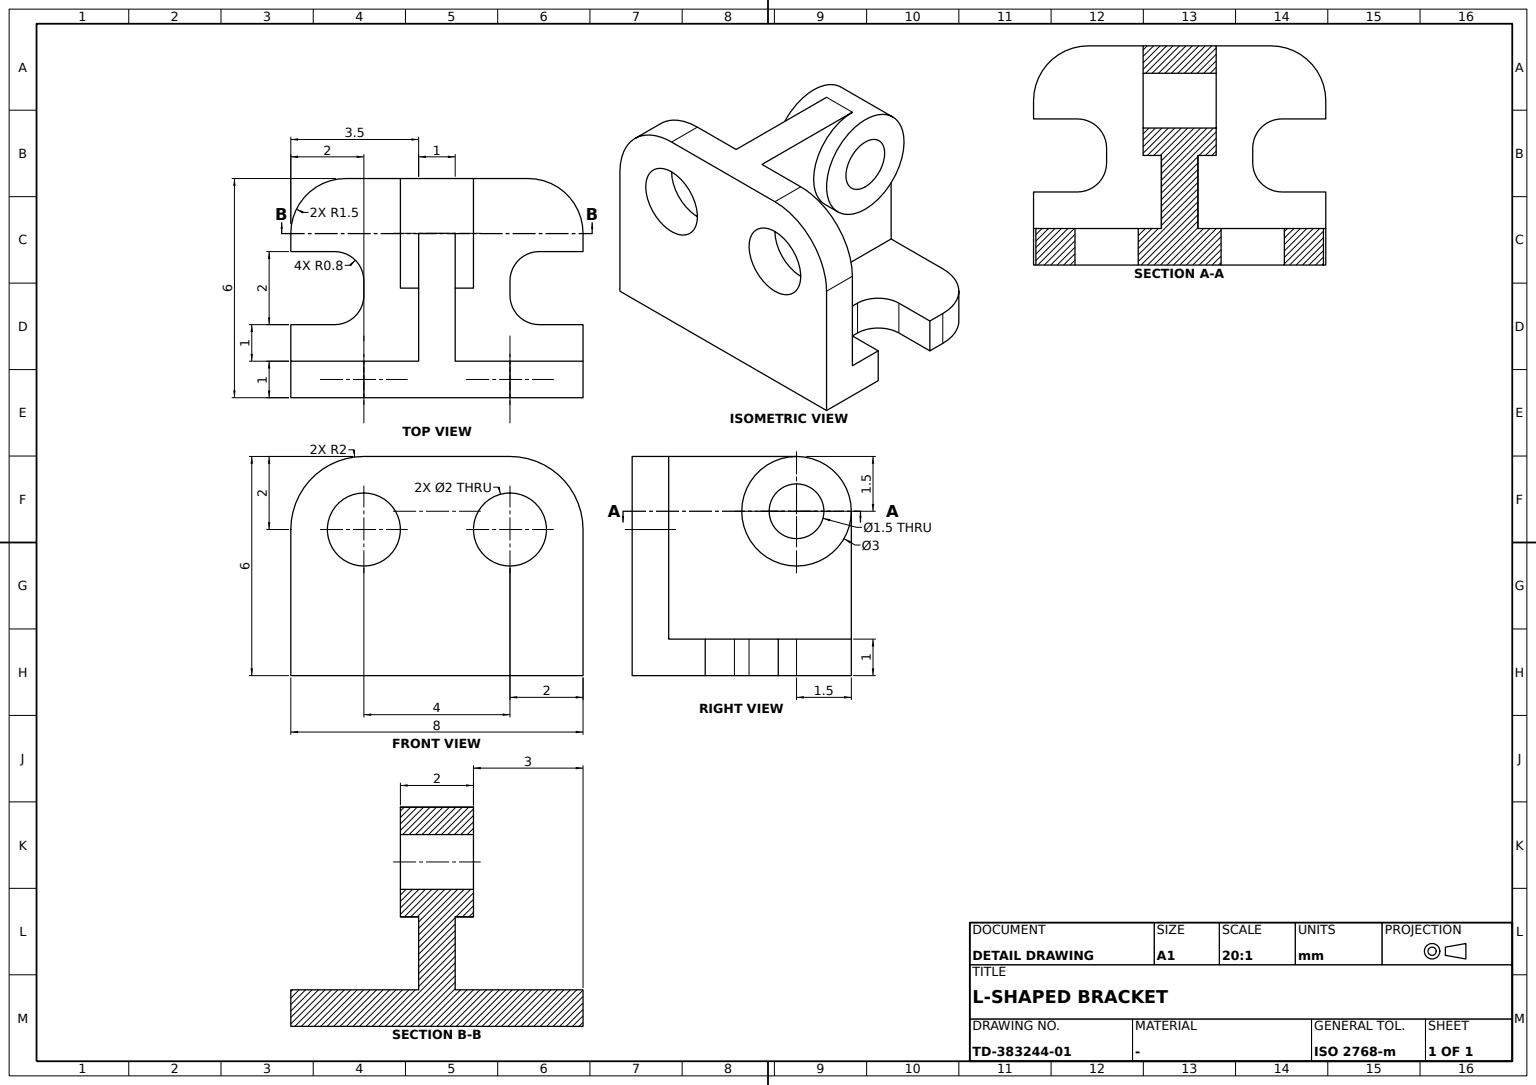
ISO-10303-21;
HEADER;
FILE_DESCRIPTION((''),'2;1');
FILE_NAME('','',(''),(''),'','','');
FILE_SCHEMA(('AUTOMOTIVE_DESIGN'));
ENDSEC;
DATA;
#1=APPLICATION_CONTEXT('');
#2=PRODUCT_CONTEXT('',#1,'mechanical');
#3=PRODUCT('','','',(#2));
#4=PRODUCT_DEFINITION_FORMATION('','',#3);
#5=PRODUCT_DEFINITION_CONTEXT('',#1,'design');
#6=PRODUCT_DEFINITION('','',#4,#5);
#7=PRODUCT_DEFINITION_SHAPE('','',#6);
#8=(LENGTH_UNIT()NAMED_UNIT(*)SI_UNIT(.MILLI.,.METRE.));
#9=(NAMED_UNIT(*)PLANE_ANGLE_UNIT()SI_UNIT($,.RADIAN.));
#10=(NAMED_UNIT(*)SI_UNIT($,.STERADIAN.)SOLID_ANGLE_UNIT());
#11=UNCERTAINTY_MEASURE_WITH_UNIT(LENGTH_MEASURE(0.005),#8,'distance_accuracy_value','');
#12=(GEOMETRIC_REPRESENTATION_CONTEXT(3)GLOBAL_UNCERTAINTY_ASSIGNED_CONTEXT((#11))GLOBAL_UNIT_ASSIGNED_CONTEXT((#8,#9,#10))REPRESENTATION_CONTEXT('',''));
#13=CARTESIAN_POINT('',(-2.,0.2,0.));
#14=VERTEX_POINT('',#13);
#15=CARTESIAN_POINT('',(-2.,-0.2,0.));
#16=VERTEX_POINT('',#15);
#17=CARTESIAN_POINT('',(-2.,0.,0.));
#18=DIRECTION('',(0.,-1.,0.));
#19=VECTOR('',#18,1000.);
#20=LINE('',#17,#19);
#21=EDGE_CURVE('',#14,#16,#20,.T.);
#22=ORIENTED_EDGE('',*,*,#21,.T.);
#23=CARTESIAN_POINT('',(-2.,-0.2,1.));
#24=VERTEX_POINT('',#23);
#25=CARTESIAN_POINT('',(-2.,-0.2,0.5));
#26=DIRECTION('',(0.,0.,1.));
#27=VECTOR('',#26,1000.);
#28=LINE('',#25,#27);
#29=EDGE_CURVE('',#16,#24,#28,.T.);
#30=ORIENTED_EDGE('',*,*,#29,.T.);
#31=CARTESIAN_POINT('',(-2.,0.2,1.));
#32=VERTEX_POINT('',#31);
#33=CARTESIAN_POINT('',(-2.,0.,1.));
#34=LINE('',#33,#19);
#35=EDGE_CURVE('',#32,#24,#34,.T.);
#36=ORIENTED_EDGE('',*,*,#35,.F.);
#37=CARTESIAN_POINT('',(-2.,0.2,0.5));
#38=LINE('',#37,#27);
#39=EDGE_CURVE('',#14,#32,#38,.T.);
#40=ORIENTED_EDGE('',*,*,#39,.F.);
#41=EDGE_LOOP('',(#22,#30,#36,#40));
#42=FACE_BOUND('',#41,.T.);
#43=DIRECTION('',(-1.,0.,0.));
#44=AXIS2_PLACEMENT_3D('',#13,#43,#18);
#45=PLANE('',#44);
#46=ADVANCED_FACE('',(#42),#45,.T.);
#47=CARTESIAN_POINT('',(2.8,1.,0.));
#48=VERTEX_POINT('',#47);
#49=CARTESIAN_POINT('',(2.8,1.,1.));
#50=VERTEX_POINT('',#49);
#51=CARTESIAN_POINT('',(2.8,1.,0.5));
#52=LINE('',#51,#27);
#53=EDGE_CURVE('',#48,#50,#52,.T.);
#54=ORIENTED_EDGE('',*,*,#53,.F.);
#55=CARTESIAN_POINT('',(4.,1.,0.));
#56=VERTEX_POINT('',#55);
#57=CARTESIAN_POINT('',(-2.8,1.,0.));
#58=DIRECTION('',(1.,0.,0.));
#59=VECTOR('',#58,1000.);
#60=LINE('',#57,#59);
#61=EDGE_CURVE('',#48,#56,#60,.T.);
#62=ORIENTED_EDGE('',*,*,#61,.T.);
#63=CARTESIAN_POINT('',(4.,1.,1.));
#64=VERTEX_POINT('',#63);
#65=LINE('',#55,#27);
#66=EDGE_CURVE('',#56,#64,#65,.T.);
#67=ORIENTED_EDGE('',*,*,#66,.T.);
#68=CARTESIAN_POINT('',(-2.8,1.,1.));
#69=LINE('',#68,#59);
#70=EDGE_CURVE('',#50,#64,#69,.T.);
#71=ORIENTED_EDGE('',*,*,#70,.F.);
#72=EDGE_LOOP('',(#54,#62,#67,#71));
#73=FACE_BOUND('',#72,.T.);
#74=DIRECTION('',(0.,1.,0.));
#75=AXIS2_PLACEMENT_3D('',#57,#74,#43);
#76=PLANE('',#75);
#77=ADVANCED_FACE('',(#73),#76,.F.);
#78=CARTESIAN_POINT('',(0.5,3.,1.));
#79=VERTEX_POINT('',#78);
#80=CARTESIAN_POINT('',(0.5,3.,4.5));
#81=VERTEX_POINT('',#80);
#82=CARTESIAN_POINT('',(0.5,3.,0.));
#83=LINE('',#82,#27);
#84=EDGE_CURVE('',#79,#81,#83,.T.);
#85=ORIENTED_EDGE('',*,*,#84,.F.);
#86=CARTESIAN_POINT('',(2.5,3.,1.));
#87=VERTEX_POINT('',#86);
#88=CARTESIAN_POINT('',(0.,3.,1.));
#89=LINE('',#88,#59);
#90=EDGE_CURVE('',#79,#87,#89,.T.);
#91=ORIENTED_EDGE('',*,*,#90,.T.);
#92=CARTESIAN_POINT('',(2.5,3.,0.));
#93=VERTEX_POINT('',#92);
#94=CARTESIAN_POINT('',(2.5,3.,0.5));
#95=LINE('',#94,#27);
#96=EDGE_CURVE('',#93,#87,#95,.T.);
#97=ORIENTED_EDGE('',*,*,#96,.F.);
#98=CARTESIAN_POINT('',(-2.5,3.,0.));
#99=VERTEX_POINT('',#98);
#100=CARTESIAN_POINT('',(0.,3.,0.));
#101=LINE('',#100,#59);
#102=EDGE_CURVE('',#99,#93,#101,.T.);
#103=ORIENTED_EDGE('',*,*,#102,.F.);
#104=CARTESIAN_POINT('',(-2.5,3.,1.));
#105=VERTEX_POINT('',#104);
#106=CARTESIAN_POINT('',(-2.5,3.,0.5));
#107=LINE('',#106,#27);
#108=EDGE_CURVE('',#99,#105,#107,.T.);
#109=ORIENTED_EDGE('',*,*,#108,.T.);
#110=CARTESIAN_POINT('',(-0.5,3.,1.));
#111=VERTEX_POINT('',#110);
#112=EDGE_CURVE('',#105,#111,#89,.T.);
#113=ORIENTED_EDGE('',*,*,#112,.T.);
#114=CARTESIAN_POINT('',(-0.5,3.,4.5));
#115=VERTEX_POINT('',#114);
#116=CARTESIAN_POINT('',(-0.5,3.,0.));
#117=LINE('',#116,#27);
#118=EDGE_CURVE('',#111,#115,#117,.T.);
#119=ORIENTED_EDGE('',*,*,#118,.T.);
#120=CARTESIAN_POINT('',(0.,3.,4.5));
#121=LINE('',#120,#59);
#122=EDGE_CURVE('',#115,#81,#121,.T.);
#123=ORIENTED_EDGE('',*,*,#122,.T.);
#124=EDGE_LOOP('',(#85,#91,#97,#103,#109,#113,#119,#123));
#125=FACE_BOUND('',#124,.T.);
#126=AXIS2_PLACEMENT_3D('',#98,#18,#58);
#127=PLANE('',#126);
#128=ADVANCED_FACE('',(#125),#127,.F.);
#129=CARTESIAN_POINT('',(-2.8,-1.,0.));
#130=VERTEX_POINT('',#129);
#131=CARTESIAN_POINT('',(-4.,-1.,0.));
#132=VERTEX_POINT('',#131);
#133=CARTESIAN_POINT('',(0.,-1.,0.));
#134=VECTOR('',#43,1000.);
#135=LINE('',#133,#134);
#136=EDGE_CURVE('',#130,#132,#135,.T.);
#137=ORIENTED_EDGE('',*,*,#136,.F.);
#138=CARTESIAN_POINT('',(-2.8,-0.2,0.));
#139=AXIS2_PLACEMENT_3D('',#138,#26,#58);
#140=CIRCLE('',#139,0.8);
#141=EDGE_CURVE('',#130,#16,#140,.T.);
#142=ORIENTED_EDGE('',*,*,#141,.T.);
#143=ORIENTED_EDGE('',*,*,#21,.F.);
#144=VERTEX_POINT('',#57);
#145=CARTESIAN_POINT('',(-2.8,0.2,0.));
#146=AXIS2_PLACEMENT_3D('',#145,#26,#58);
#147=CIRCLE('',#146,0.8);
#148=EDGE_CURVE('',#14,#144,#147,.T.);
#149=ORIENTED_EDGE('',*,*,#148,.T.);
#150=CARTESIAN_POINT('',(-4.,1.,0.));
#151=VERTEX_POINT('',#150);
#152=CARTESIAN_POINT('',(0.,1.,0.));
#153=LINE('',#152,#134);
#154=EDGE_CURVE('',#144,#151,#153,.T.);
#155=ORIENTED_EDGE('',*,*,#154,.T.);
#156=CARTESIAN_POINT('',(-4.,1.5,0.));
#157=VERTEX_POINT('',#156);
#158=CARTESIAN_POINT('',(-4.,0.,0.));
#159=VECTOR('',#74,1000.);
#160=LINE('',#158,#159);
#161=EDGE_CURVE('',#151,#157,#160,.T.);
#162=ORIENTED_EDGE('',*,*,#161,.T.);
#163=CARTESIAN_POINT('',(-2.5,1.5,0.));
#164=AXIS2_PLACEMENT_3D('',#163,#26,#58);
#165=CIRCLE('',#164,1.5);
#166=EDGE_CURVE('',#99,#157,#165,.T.);
#167=ORIENTED_EDGE('',*,*,#166,.F.);
#168=ORIENTED_EDGE('',*,*,#102,.T.);
#169=CARTESIAN_POINT('',(4.,1.5,0.));
#170=VERTEX_POINT('',#169);
#171=CARTESIAN_POINT('',(2.5,1.5,0.));
#172=AXIS2_PLACEMENT_3D('',#171,#26,#58);
#173=CIRCLE('',#172,1.5);
#174=EDGE_CURVE('',#170,#93,#173,.T.);
#175=ORIENTED_EDGE('',*,*,#174,.F.);
#176=CARTESIAN_POINT('',(4.,0.,0.));
#177=LINE('',#176,#19);
#178=EDGE_CURVE('',#170,#56,#177,.T.);
#179=ORIENTED_EDGE('',*,*,#178,.T.);
#180=ORIENTED_EDGE('',*,*,#61,.F.);
#181=CARTESIAN_POINT('',(2.,0.2,0.));
#182=VERTEX_POINT('',#181);
#183=CARTESIAN_POINT('',(2.8,0.2,0.));
#184=AXIS2_PLACEMENT_3D('',#183,#26,#58);
#185=CIRCLE('',#184,0.8);
#186=EDGE_CURVE('',#48,#182,#185,.T.);
#187=ORIENTED_EDGE('',*,*,#186,.T.);
#188=CARTESIAN_POINT('',(2.,-0.2,0.));
#189=VERTEX_POINT('',#188);
#190=CARTESIAN_POINT('',(2.,0.,0.));
#191=LINE('',#190,#19);
#192=EDGE_CURVE('',#182,#189,#191,.T.);
#193=ORIENTED_EDGE('',*,*,#192,.T.);
#194=CARTESIAN_POINT('',(2.8,-1.,0.));
#195=VERTEX_POINT('',#194);
#196=CARTESIAN_POINT('',(2.8,-0.2,0.));
#197=AXIS2_PLACEMENT_3D('',#196,#26,#58);
#198=CIRCLE('',#197,0.8);
#199=EDGE_CURVE('',#189,#195,#198,.T.);
#200=ORIENTED_EDGE('',*,*,#199,.T.);
#201=CARTESIAN_POINT('',(4.,-1.,0.));
#202=VERTEX_POINT('',#201);
#203=LINE('',#129,#59);
#204=EDGE_CURVE('',#195,#202,#203,.T.);
#205=ORIENTED_EDGE('',*,*,#204,.T.);
#206=CARTESIAN_POINT('',(4.,-3.,0.));
#207=VERTEX_POINT('',#206);
#208=EDGE_CURVE('',#202,#207,#177,.T.);
#209=ORIENTED_EDGE('',*,*,#208,.T.);
#210=CARTESIAN_POINT('',(-4.,-3.,0.));
#211=VERTEX_POINT('',#210);
#212=CARTESIAN_POINT('',(0.,-3.,0.));
#213=LINE('',#212,#134);
#214=EDGE_CURVE('',#207,#211,#213,.T.);
#215=ORIENTED_EDGE('',*,*,#214,.T.);
#216=EDGE_CURVE('',#211,#132,#160,.T.);
#217=ORIENTED_EDGE('',*,*,#216,.T.);
#218=EDGE_LOOP('',(#137,#142,#143,#149,#155,#162,#167,#168,#175,#179,#180,#187,#193,#200,#205,#209,#215,#217));
#219=FACE_BOUND('',#218,.T.);
#220=CARTESIAN_POINT('',(0.,0.,0.));
#221=AXIS2_PLACEMENT_3D('',#220,#26,#58);
#222=PLANE('',#221);
#223=ADVANCED_FACE('',(#219),#222,.F.);
#224=CARTESIAN_POINT('',(4.,1.5,1.));
#225=VERTEX_POINT('',#224);
#226=CARTESIAN_POINT('',(2.5,1.5,1.));
#227=AXIS2_PLACEMENT_3D('',#226,#26,#58);
#228=CIRCLE('',#227,1.5);
#229=EDGE_CURVE('',#225,#87,#228,.T.);
#230=ORIENTED_EDGE('',*,*,#229,.F.);
#231=CARTESIAN_POINT('',(4.,1.5,0.5));
#232=LINE('',#231,#27);
#233=EDGE_CURVE('',#170,#225,#232,.T.);
#234=ORIENTED_EDGE('',*,*,#233,.F.);
#235=ORIENTED_EDGE('',*,*,#174,.T.);
#236=ORIENTED_EDGE('',*,*,#96,.T.);
#237=EDGE_LOOP('',(#230,#234,#235,#236));
#238=FACE_BOUND('',#237,.T.);
#239=CARTESIAN_POINT('',(2.5,1.5,0.5));
#240=AXIS2_PLACEMENT_3D('',#239,#26,#58);
#241=CYLINDRICAL_SURFACE('',#240,1.5);
#242=ADVANCED_FACE('',(#238),#241,.T.);
#243=CARTESIAN_POINT('',(-1.,1.5,3.));
#244=VERTEX_POINT('',#243);
#245=CARTESIAN_POINT('',(-1.,1.5,4.5));
#246=DIRECTION('',(0.,0.,-1.));
#247=AXIS2_PLACEMENT_3D('',#245,#58,#246);
#248=CIRCLE('',#247,1.5);
#249=EDGE_CURVE('',#244,#244,#248,.T.);
#250=ORIENTED_EDGE('',*,*,#249,.F.);
#251=EDGE_LOOP('',(#250));
#252=FACE_BOUND('',#251,.T.);
#253=CARTESIAN_POINT('',(-1.,1.5,3.75));
#254=VERTEX_POINT('',#253);
#255=CIRCLE('',#247,0.75);
#256=EDGE_CURVE('',#254,#254,#255,.T.);
#257=ORIENTED_EDGE('',*,*,#256,.T.);
#258=EDGE_LOOP('',(#257));
#259=FACE_BOUND('',#258,.T.);
#260=CARTESIAN_POINT('',(-1.,0.,0.));
#261=AXIS2_PLACEMENT_3D('',#260,#58,#74);
#262=PLANE('',#261);
#263=ADVANCED_FACE('',(#252,#259),#262,.F.);
#264=CARTESIAN_POINT('',(4.,-3.,4.));
#265=VERTEX_POINT('',#264);
#266=CARTESIAN_POINT('',(4.,-2.,4.));
#267=VERTEX_POINT('',#266);
#268=CARTESIAN_POINT('',(4.,-2.5,4.));
#269=LINE('',#268,#19);
#270=EDGE_CURVE('',#265,#267,#269,.F.);
#271=ORIENTED_EDGE('',*,*,#270,.F.);
#272=LINE('',#206,#27);
#273=EDGE_CURVE('',#207,#265,#272,.T.);
#274=ORIENTED_EDGE('',*,*,#273,.F.);
#275=ORIENTED_EDGE('',*,*,#208,.F.);
#276=CARTESIAN_POINT('',(4.,-1.,1.));
#277=VERTEX_POINT('',#276);
#278=LINE('',#201,#27);
#279=EDGE_CURVE('',#202,#277,#278,.T.);
#280=ORIENTED_EDGE('',*,*,#279,.T.);
#281=CARTESIAN_POINT('',(4.,-2.,1.));
#282=VERTEX_POINT('',#281);
#283=CARTESIAN_POINT('',(4.,0.,1.));
#284=LINE('',#283,#19);
#285=EDGE_CURVE('',#277,#282,#284,.T.);
#286=ORIENTED_EDGE('',*,*,#285,.T.);
#287=CARTESIAN_POINT('',(4.,-2.,0.));
#288=VECTOR('',#246,1000.);
#289=LINE('',#287,#288);
#290=EDGE_CURVE('',#267,#282,#289,.T.);
#291=ORIENTED_EDGE('',*,*,#290,.F.);
#292=EDGE_LOOP('',(#271,#274,#275,#280,#286,#291));
#293=FACE_BOUND('',#292,.T.);
#294=AXIS2_PLACEMENT_3D('',#201,#43,#18);
#295=PLANE('',#294);
#296=ADVANCED_FACE('',(#293),#295,.F.);
#297=VERTEX_POINT('',#68);
#298=CARTESIAN_POINT('',(-2.8,0.2,1.));
#299=AXIS2_PLACEMENT_3D('',#298,#26,#58);
#300=CIRCLE('',#299,0.8);
#301=EDGE_CURVE('',#32,#297,#300,.T.);
#302=ORIENTED_EDGE('',*,*,#301,.T.);
#303=CARTESIAN_POINT('',(-2.8,1.,0.5));
#304=LINE('',#303,#27);
#305=EDGE_CURVE('',#144,#297,#304,.T.);
#306=ORIENTED_EDGE('',*,*,#305,.F.);
#307=ORIENTED_EDGE('',*,*,#148,.F.);
#308=ORIENTED_EDGE('',*,*,#39,.T.);
#309=EDGE_LOOP('',(#302,#306,#307,#308));
#310=FACE_BOUND('',#309,.T.);
#311=CARTESIAN_POINT('',(-2.8,0.2,0.5));
#312=AXIS2_PLACEMENT_3D('',#311,#26,#58);
#313=CYLINDRICAL_SURFACE('',#312,0.8);
#314=ADVANCED_FACE('',(#310),#313,.F.);
#315=CARTESIAN_POINT('',(0.5,-2.,1.));
#316=VERTEX_POINT('',#315);
#317=CARTESIAN_POINT('',(0.,-2.,1.));
#318=LINE('',#317,#134);
#319=EDGE_CURVE('',#282,#316,#318,.T.);
#320=ORIENTED_EDGE('',*,*,#319,.F.);
#321=ORIENTED_EDGE('',*,*,#285,.F.);
#322=CARTESIAN_POINT('',(2.8,-1.,1.));
#323=VERTEX_POINT('',#322);
#324=CARTESIAN_POINT('',(-2.8,-1.,1.));
#325=LINE('',#324,#59);
#326=EDGE_CURVE('',#323,#277,#325,.T.);
#327=ORIENTED_EDGE('',*,*,#326,.F.);
#328=CARTESIAN_POINT('',(2.,-0.2,1.));
#329=VERTEX_POINT('',#328);
#330=CARTESIAN_POINT('',(2.8,-0.2,1.));
#331=AXIS2_PLACEMENT_3D('',#330,#26,#58);
#332=CIRCLE('',#331,0.8);
#333=EDGE_CURVE('',#329,#323,#332,.T.);
#334=ORIENTED_EDGE('',*,*,#333,.F.);
#335=CARTESIAN_POINT('',(2.,0.2,1.));
#336=VERTEX_POINT('',#335);
#337=CARTESIAN_POINT('',(2.,0.,1.));
#338=LINE('',#337,#19);
#339=EDGE_CURVE('',#336,#329,#338,.T.);
#340=ORIENTED_EDGE('',*,*,#339,.F.);
#341=CARTESIAN_POINT('',(2.8,0.2,1.));
#342=AXIS2_PLACEMENT_3D('',#341,#26,#58);
#343=CIRCLE('',#342,0.8);
#344=EDGE_CURVE('',#50,#336,#343,.T.);
#345=ORIENTED_EDGE('',*,*,#344,.F.);
#346=ORIENTED_EDGE('',*,*,#70,.T.);
#347=EDGE_CURVE('',#225,#64,#284,.T.);
#348=ORIENTED_EDGE('',*,*,#347,.F.);
#349=ORIENTED_EDGE('',*,*,#229,.T.);
#350=ORIENTED_EDGE('',*,*,#90,.F.);
#351=CARTESIAN_POINT('',(0.5,0.,1.));
#352=LINE('',#351,#159);
#353=EDGE_CURVE('',#316,#79,#352,.T.);
#354=ORIENTED_EDGE('',*,*,#353,.F.);
#355=EDGE_LOOP('',(#320,#321,#327,#334,#340,#345,#346,#348,#349,#350,#354));
#356=FACE_BOUND('',#355,.T.);
#357=CARTESIAN_POINT('',(0.,0.,1.));
#358=AXIS2_PLACEMENT_3D('',#357,#26,#58);
#359=PLANE('',#358);
#360=ADVANCED_FACE('',(#356),#359,.T.);
#361=CARTESIAN_POINT('',(2.,-3.,5.));
#362=VERTEX_POINT('',#361);
#363=CARTESIAN_POINT('',(2.,-3.,4.));
#364=AXIS2_PLACEMENT_3D('',#363,#74,#26);
#365=CIRCLE('',#364,1.);
#366=EDGE_CURVE('',#362,#362,#365,.T.);
#367=ORIENTED_EDGE('',*,*,#366,.F.);
#368=EDGE_LOOP('',(#367));
#369=FACE_BOUND('',#368,.T.);
#370=CARTESIAN_POINT('',(2.,-2.,3.));
#371=VERTEX_POINT('',#370);
#372=CARTESIAN_POINT('',(2.,-2.,4.));
#373=AXIS2_PLACEMENT_3D('',#372,#18,#246);
#374=CIRCLE('',#373,1.);
#375=EDGE_CURVE('',#371,#371,#374,.F.);
#376=ORIENTED_EDGE('',*,*,#375,.T.);
#377=EDGE_LOOP('',(#376));
#378=FACE_BOUND('',#377,.T.);
#379=CARTESIAN_POINT('',(2.,-2.5,4.));
#380=AXIS2_PLACEMENT_3D('',#379,#74,#43);
#381=CYLINDRICAL_SURFACE('',#380,1.);
#382=ADVANCED_FACE('',(#369,#378),#381,.F.);
#383=ORIENTED_EDGE('',*,*,#326,.T.);
#384=ORIENTED_EDGE('',*,*,#279,.F.);
#385=ORIENTED_EDGE('',*,*,#204,.F.);
#386=CARTESIAN_POINT('',(2.8,-1.,0.5));
#387=LINE('',#386,#27);
#388=EDGE_CURVE('',#195,#323,#387,.T.);
#389=ORIENTED_EDGE('',*,*,#388,.T.);
#390=EDGE_LOOP('',(#383,#384,#385,#389));
#391=FACE_BOUND('',#390,.T.);
#392=AXIS2_PLACEMENT_3D('',#129,#74,#43);
#393=PLANE('',#392);
#394=ADVANCED_FACE('',(#391),#393,.T.);
#395=CARTESIAN_POINT('',(-4.,1.5,1.));
#396=VERTEX_POINT('',#395);
#397=CARTESIAN_POINT('',(-2.5,1.5,1.));
#398=AXIS2_PLACEMENT_3D('',#397,#26,#58);
#399=CIRCLE('',#398,1.5);
#400=EDGE_CURVE('',#105,#396,#399,.T.);
#401=ORIENTED_EDGE('',*,*,#400,.F.);
#402=ORIENTED_EDGE('',*,*,#108,.F.);
#403=ORIENTED_EDGE('',*,*,#166,.T.);
#404=CARTESIAN_POINT('',(-4.,1.5,0.5));
#405=LINE('',#404,#27);
#406=EDGE_CURVE('',#157,#396,#405,.T.);
#407=ORIENTED_EDGE('',*,*,#406,.T.);
#408=EDGE_LOOP('',(#401,#402,#403,#407));
#409=FACE_BOUND('',#408,.T.);
#410=CARTESIAN_POINT('',(-2.5,1.5,0.5));
#411=AXIS2_PLACEMENT_3D('',#410,#26,#58);
#412=CYLINDRICAL_SURFACE('',#411,1.5);
#413=ADVANCED_FACE('',(#409),#412,.T.);
#414=ORIENTED_EDGE('',*,*,#353,.T.);
#415=ORIENTED_EDGE('',*,*,#84,.T.);
#416=CARTESIAN_POINT('',(0.5,1.5,6.));
#417=VERTEX_POINT('',#416);
#418=CARTESIAN_POINT('',(0.5,1.5,4.5));
#419=AXIS2_PLACEMENT_3D('',#418,#58,#246);
#420=CIRCLE('',#419,1.5);
#421=EDGE_CURVE('',#417,#81,#420,.T.);
#422=ORIENTED_EDGE('',*,*,#421,.F.);
#423=CARTESIAN_POINT('',(0.5,-2.,6.));
#424=VERTEX_POINT('',#423);
#425=CARTESIAN_POINT('',(0.5,-3.,6.));
#426=LINE('',#425,#159);
#427=EDGE_CURVE('',#424,#417,#426,.T.);
#428=ORIENTED_EDGE('',*,*,#427,.F.);
#429=CARTESIAN_POINT('',(0.5,-2.,0.));
#430=LINE('',#429,#288);
#431=EDGE_CURVE('',#424,#316,#430,.T.);
#432=ORIENTED_EDGE('',*,*,#431,.T.);
#433=EDGE_LOOP('',(#414,#415,#422,#428,#432));
#434=FACE_BOUND('',#433,.T.);
#435=CARTESIAN_POINT('',(0.5,0.,0.));
#436=AXIS2_PLACEMENT_3D('',#435,#58,#74);
#437=PLANE('',#436);
#438=ADVANCED_FACE('',(#434),#437,.T.);
#439=CARTESIAN_POINT('',(-2.,-3.,5.));
#440=VERTEX_POINT('',#439);
#441=CARTESIAN_POINT('',(-2.,-3.,4.));
#442=AXIS2_PLACEMENT_3D('',#441,#74,#26);
#443=CIRCLE('',#442,1.);
#444=EDGE_CURVE('',#440,#440,#443,.T.);
#445=ORIENTED_EDGE('',*,*,#444,.T.);
#446=EDGE_LOOP('',(#445));
#447=FACE_BOUND('',#446,.T.);
#448=ORIENTED_EDGE('',*,*,#366,.T.);
#449=EDGE_LOOP('',(#448));
#450=FACE_BOUND('',#449,.T.);
#451=ORIENTED_EDGE('',*,*,#273,.T.);
#452=CARTESIAN_POINT('',(2.,-3.,6.));
#453=VERTEX_POINT('',#452);
#454=CIRCLE('',#364,2.);
#455=EDGE_CURVE('',#265,#453,#454,.F.);
#456=ORIENTED_EDGE('',*,*,#455,.T.);
#457=CARTESIAN_POINT('',(-2.,-3.,6.));
#458=VERTEX_POINT('',#457);
#459=CARTESIAN_POINT('',(4.,-3.,6.));
#460=LINE('',#459,#59);
#461=EDGE_CURVE('',#458,#453,#460,.T.);
#462=ORIENTED_EDGE('',*,*,#461,.F.);
#463=CARTESIAN_POINT('',(-4.,-3.,4.));
#464=VERTEX_POINT('',#463);
#465=CIRCLE('',#442,2.);
#466=EDGE_CURVE('',#458,#464,#465,.F.);
#467=ORIENTED_EDGE('',*,*,#466,.T.);
#468=LINE('',#210,#27);
#469=EDGE_CURVE('',#211,#464,#468,.T.);
#470=ORIENTED_EDGE('',*,*,#469,.F.);
#471=ORIENTED_EDGE('',*,*,#214,.F.);
#472=EDGE_LOOP('',(#451,#456,#462,#467,#470,#471));
#473=FACE_BOUND('',#472,.T.);
#474=AXIS2_PLACEMENT_3D('',#206,#74,#43);
#475=PLANE('',#474);
#476=ADVANCED_FACE('',(#447,#450,#473),#475,.F.);
#477=ORIENTED_EDGE('',*,*,#29,.F.);
#478=ORIENTED_EDGE('',*,*,#141,.F.);
#479=VERTEX_POINT('',#324);
#480=CARTESIAN_POINT('',(-2.8,-1.,0.5));
#481=LINE('',#480,#27);
#482=EDGE_CURVE('',#130,#479,#481,.T.);
#483=ORIENTED_EDGE('',*,*,#482,.T.);
#484=CARTESIAN_POINT('',(-2.8,-0.2,1.));
#485=AXIS2_PLACEMENT_3D('',#484,#26,#58);
#486=CIRCLE('',#485,0.8);
#487=EDGE_CURVE('',#479,#24,#486,.T.);
#488=ORIENTED_EDGE('',*,*,#487,.T.);
#489=EDGE_LOOP('',(#477,#478,#483,#488));
#490=FACE_BOUND('',#489,.T.);
#491=CARTESIAN_POINT('',(-2.8,-0.2,0.5));
#492=AXIS2_PLACEMENT_3D('',#491,#26,#58);
#493=CYLINDRICAL_SURFACE('',#492,0.8);
#494=ADVANCED_FACE('',(#490),#493,.F.);
#495=ORIENTED_EDGE('',*,*,#270,.T.);
#496=CARTESIAN_POINT('',(2.,-2.,6.));
#497=VERTEX_POINT('',#496);
#498=CIRCLE('',#373,2.);
#499=EDGE_CURVE('',#267,#497,#498,.T.);
#500=ORIENTED_EDGE('',*,*,#499,.T.);
#501=CARTESIAN_POINT('',(2.,-2.5,6.));
#502=LINE('',#501,#19);
#503=EDGE_CURVE('',#453,#497,#502,.F.);
#504=ORIENTED_EDGE('',*,*,#503,.F.);
#505=ORIENTED_EDGE('',*,*,#455,.F.);
#506=EDGE_LOOP('',(#495,#500,#504,#505));
#507=FACE_BOUND('',#506,.T.);
#508=AXIS2_PLACEMENT_3D('',#379,#18,#58);
#509=CYLINDRICAL_SURFACE('',#508,2.);
#510=ADVANCED_FACE('',(#507),#509,.T.);
#511=ORIENTED_EDGE('',*,*,#344,.T.);
#512=CARTESIAN_POINT('',(2.,0.2,0.5));
#513=LINE('',#512,#27);
#514=EDGE_CURVE('',#182,#336,#513,.T.);
#515=ORIENTED_EDGE('',*,*,#514,.F.);
#516=ORIENTED_EDGE('',*,*,#186,.F.);
#517=ORIENTED_EDGE('',*,*,#53,.T.);
#518=EDGE_LOOP('',(#511,#515,#516,#517));
#519=FACE_BOUND('',#518,.T.);
#520=CARTESIAN_POINT('',(2.8,0.2,0.5));
#521=AXIS2_PLACEMENT_3D('',#520,#26,#58);
#522=CYLINDRICAL_SURFACE('',#521,0.8);
#523=ADVANCED_FACE('',(#519),#522,.F.);
#524=CARTESIAN_POINT('',(-0.5,1.5,6.));
#525=VERTEX_POINT('',#524);
#526=CARTESIAN_POINT('',(0.,1.5,6.));
#527=LINE('',#526,#59);
#528=EDGE_CURVE('',#525,#417,#527,.T.);
#529=ORIENTED_EDGE('',*,*,#528,.T.);
#530=ORIENTED_EDGE('',*,*,#421,.T.);
#531=ORIENTED_EDGE('',*,*,#122,.F.);
#532=CARTESIAN_POINT('',(-0.5,1.5,4.5));
#533=AXIS2_PLACEMENT_3D('',#532,#58,#246);
#534=CIRCLE('',#533,1.5);
#535=EDGE_CURVE('',#525,#115,#534,.T.);
#536=ORIENTED_EDGE('',*,*,#535,.F.);
#537=EDGE_LOOP('',(#529,#530,#531,#536));
#538=FACE_BOUND('',#537,.T.);
#539=CARTESIAN_POINT('',(1.,1.5,3.));
#540=VERTEX_POINT('',#539);
#541=CARTESIAN_POINT('',(1.,1.5,4.5));
#542=AXIS2_PLACEMENT_3D('',#541,#58,#246);
#543=CIRCLE('',#542,1.5);
#544=EDGE_CURVE('',#540,#540,#543,.T.);
#545=ORIENTED_EDGE('',*,*,#544,.F.);
#546=EDGE_LOOP('',(#545));
#547=FACE_BOUND('',#546,.T.);
#548=ORIENTED_EDGE('',*,*,#249,.T.);
#549=EDGE_LOOP('',(#548));
#550=FACE_BOUND('',#549,.T.);
#551=CARTESIAN_POINT('',(0.,1.5,4.5));
#552=AXIS2_PLACEMENT_3D('',#551,#58,#74);
#553=CYLINDRICAL_SURFACE('',#552,1.5);
#554=ADVANCED_FACE('',(#538,#547,#550),#553,.T.);
#555=ORIENTED_EDGE('',*,*,#136,.T.);
#556=CARTESIAN_POINT('',(-4.,-1.,1.));
#557=VERTEX_POINT('',#556);
#558=LINE('',#131,#27);
#559=EDGE_CURVE('',#132,#557,#558,.T.);
#560=ORIENTED_EDGE('',*,*,#559,.T.);
#561=CARTESIAN_POINT('',(0.,-1.,1.));
#562=LINE('',#561,#134);
#563=EDGE_CURVE('',#479,#557,#562,.T.);
#564=ORIENTED_EDGE('',*,*,#563,.F.);
#565=ORIENTED_EDGE('',*,*,#482,.F.);
#566=EDGE_LOOP('',(#555,#560,#564,#565));
#567=FACE_BOUND('',#566,.T.);
#568=ADVANCED_FACE('',(#567),#393,.T.);
#569=ORIENTED_EDGE('',*,*,#154,.F.);
#570=ORIENTED_EDGE('',*,*,#305,.T.);
#571=CARTESIAN_POINT('',(-4.,1.,1.));
#572=VERTEX_POINT('',#571);
#573=CARTESIAN_POINT('',(0.,1.,1.));
#574=LINE('',#573,#134);
#575=EDGE_CURVE('',#297,#572,#574,.T.);
#576=ORIENTED_EDGE('',*,*,#575,.T.);
#577=LINE('',#150,#27);
#578=EDGE_CURVE('',#151,#572,#577,.T.);
#579=ORIENTED_EDGE('',*,*,#578,.F.);
#580=EDGE_LOOP('',(#569,#570,#576,#579));
#581=FACE_BOUND('',#580,.T.);
#582=ADVANCED_FACE('',(#581),#76,.F.);
#583=ORIENTED_EDGE('',*,*,#544,.T.);
#584=EDGE_LOOP('',(#583));
#585=FACE_BOUND('',#584,.T.);
#586=CARTESIAN_POINT('',(1.,1.5,3.75));
#587=VERTEX_POINT('',#586);
#588=CIRCLE('',#542,0.75);
#589=EDGE_CURVE('',#587,#587,#588,.T.);
#590=ORIENTED_EDGE('',*,*,#589,.F.);
#591=EDGE_LOOP('',(#590));
#592=FACE_BOUND('',#591,.T.);
#593=CARTESIAN_POINT('',(1.,0.,0.));
#594=AXIS2_PLACEMENT_3D('',#593,#58,#74);
#595=PLANE('',#594);
#596=ADVANCED_FACE('',(#585,#592),#595,.T.);
#597=ORIENTED_EDGE('',*,*,#118,.F.);
#598=CARTESIAN_POINT('',(-0.5,-2.,1.));
#599=VERTEX_POINT('',#598);
#600=CARTESIAN_POINT('',(-0.5,0.,1.));
#601=LINE('',#600,#159);
#602=EDGE_CURVE('',#599,#111,#601,.T.);
#603=ORIENTED_EDGE('',*,*,#602,.F.);
#604=CARTESIAN_POINT('',(-0.5,-2.,6.));
#605=VERTEX_POINT('',#604);
#606=CARTESIAN_POINT('',(-0.5,-2.,0.));
#607=LINE('',#606,#288);
#608=EDGE_CURVE('',#605,#599,#607,.T.);
#609=ORIENTED_EDGE('',*,*,#608,.F.);
#610=CARTESIAN_POINT('',(-0.5,-3.,6.));
#611=LINE('',#610,#159);
#612=EDGE_CURVE('',#605,#525,#611,.T.);
#613=ORIENTED_EDGE('',*,*,#612,.T.);
#614=ORIENTED_EDGE('',*,*,#535,.T.);
#615=EDGE_LOOP('',(#597,#603,#609,#613,#614));
#616=FACE_BOUND('',#615,.T.);
#617=CARTESIAN_POINT('',(-0.5,0.,0.));
#618=AXIS2_PLACEMENT_3D('',#617,#58,#74);
#619=PLANE('',#618);
#620=ADVANCED_FACE('',(#616),#619,.F.);
#621=ORIENTED_EDGE('',*,*,#578,.T.);
#622=CARTESIAN_POINT('',(-4.,0.,1.));
#623=LINE('',#622,#159);
#624=EDGE_CURVE('',#572,#396,#623,.T.);
#625=ORIENTED_EDGE('',*,*,#624,.T.);
#626=ORIENTED_EDGE('',*,*,#406,.F.);
#627=ORIENTED_EDGE('',*,*,#161,.F.);
#628=EDGE_LOOP('',(#621,#625,#626,#627));
#629=FACE_BOUND('',#628,.T.);
#630=AXIS2_PLACEMENT_3D('',#150,#58,#74);
#631=PLANE('',#630);
#632=ADVANCED_FACE('',(#629),#631,.F.);
#633=CARTESIAN_POINT('',(-2.,-2.,6.));
#634=VERTEX_POINT('',#633);
#635=LINE('',#633,#59);
#636=EDGE_CURVE('',#634,#605,#635,.T.);
#637=ORIENTED_EDGE('',*,*,#636,.F.);
#638=CARTESIAN_POINT('',(-2.,-2.5,6.));
#639=LINE('',#638,#19);
#640=EDGE_CURVE('',#458,#634,#639,.F.);
#641=ORIENTED_EDGE('',*,*,#640,.F.);
#642=ORIENTED_EDGE('',*,*,#461,.T.);
#643=ORIENTED_EDGE('',*,*,#503,.T.);
#644=EDGE_CURVE('',#424,#497,#635,.T.);
#645=ORIENTED_EDGE('',*,*,#644,.F.);
#646=ORIENTED_EDGE('',*,*,#427,.T.);
#647=ORIENTED_EDGE('',*,*,#528,.F.);
#648=ORIENTED_EDGE('',*,*,#612,.F.);
#649=EDGE_LOOP('',(#637,#641,#642,#643,#645,#646,#647,#648));
#650=FACE_BOUND('',#649,.T.);
#651=AXIS2_PLACEMENT_3D('',#457,#26,#58);
#652=PLANE('',#651);
#653=ADVANCED_FACE('',(#650),#652,.T.);
#654=ORIENTED_EDGE('',*,*,#66,.F.);
#655=ORIENTED_EDGE('',*,*,#178,.F.);
#656=ORIENTED_EDGE('',*,*,#233,.T.);
#657=ORIENTED_EDGE('',*,*,#347,.T.);
#658=EDGE_LOOP('',(#654,#655,#656,#657));
#659=FACE_BOUND('',#658,.T.);
#660=ADVANCED_FACE('',(#659),#295,.F.);
#661=ORIENTED_EDGE('',*,*,#256,.F.);
#662=EDGE_LOOP('',(#661));
#663=FACE_BOUND('',#662,.T.);
#664=ORIENTED_EDGE('',*,*,#589,.T.);
#665=EDGE_LOOP('',(#664));
#666=FACE_BOUND('',#665,.T.);
#667=CARTESIAN_POINT('',(-2.16,1.5,4.5));
#668=AXIS2_PLACEMENT_3D('',#667,#58,#74);
#669=CYLINDRICAL_SURFACE('',#668,0.75);
#670=ADVANCED_FACE('',(#663,#666),#669,.F.);
#671=CARTESIAN_POINT('',(-4.,-2.,1.));
#672=VERTEX_POINT('',#671);
#673=EDGE_CURVE('',#599,#672,#318,.T.);
#674=ORIENTED_EDGE('',*,*,#673,.T.);
#675=CARTESIAN_POINT('',(-4.,-2.,4.));
#676=VERTEX_POINT('',#675);
#677=CARTESIAN_POINT('',(-4.,-2.,0.));
#678=LINE('',#677,#27);
#679=EDGE_CURVE('',#672,#676,#678,.T.);
#680=ORIENTED_EDGE('',*,*,#679,.T.);
#681=CARTESIAN_POINT('',(-2.,-2.,4.));
#682=AXIS2_PLACEMENT_3D('',#681,#18,#246);
#683=CIRCLE('',#682,2.);
#684=EDGE_CURVE('',#634,#676,#683,.T.);
#685=ORIENTED_EDGE('',*,*,#684,.F.);
#686=ORIENTED_EDGE('',*,*,#636,.T.);
#687=ORIENTED_EDGE('',*,*,#608,.T.);
#688=EDGE_LOOP('',(#674,#680,#685,#686,#687));
#689=FACE_BOUND('',#688,.T.);
#690=CARTESIAN_POINT('',(-2.,-2.,3.));
#691=VERTEX_POINT('',#690);
#692=CIRCLE('',#682,1.);
#693=EDGE_CURVE('',#691,#691,#692,.F.);
#694=ORIENTED_EDGE('',*,*,#693,.F.);
#695=EDGE_LOOP('',(#694));
#696=FACE_BOUND('',#695,.T.);
#697=CARTESIAN_POINT('',(0.,-2.,0.));
#698=AXIS2_PLACEMENT_3D('',#697,#18,#58);
#699=PLANE('',#698);
#700=ADVANCED_FACE('',(#689,#696),#699,.F.);
#701=ORIENTED_EDGE('',*,*,#216,.F.);
#702=ORIENTED_EDGE('',*,*,#469,.T.);
#703=CARTESIAN_POINT('',(-4.,-2.5,4.));
#704=LINE('',#703,#19);
#705=EDGE_CURVE('',#464,#676,#704,.F.);
#706=ORIENTED_EDGE('',*,*,#705,.T.);
#707=ORIENTED_EDGE('',*,*,#679,.F.);
#708=EDGE_CURVE('',#672,#557,#623,.T.);
#709=ORIENTED_EDGE('',*,*,#708,.T.);
#710=ORIENTED_EDGE('',*,*,#559,.F.);
#711=EDGE_LOOP('',(#701,#702,#706,#707,#709,#710));
#712=FACE_BOUND('',#711,.T.);
#713=ADVANCED_FACE('',(#712),#631,.F.);
#714=ORIENTED_EDGE('',*,*,#575,.F.);
#715=ORIENTED_EDGE('',*,*,#301,.F.);
#716=ORIENTED_EDGE('',*,*,#35,.T.);
#717=ORIENTED_EDGE('',*,*,#487,.F.);
#718=ORIENTED_EDGE('',*,*,#563,.T.);
#719=ORIENTED_EDGE('',*,*,#708,.F.);
#720=ORIENTED_EDGE('',*,*,#673,.F.);
#721=ORIENTED_EDGE('',*,*,#602,.T.);
#722=ORIENTED_EDGE('',*,*,#112,.F.);
#723=ORIENTED_EDGE('',*,*,#400,.T.);
#724=ORIENTED_EDGE('',*,*,#624,.F.);
#725=EDGE_LOOP('',(#714,#715,#716,#717,#718,#719,#720,#721,#722,#723,#724));
#726=FACE_BOUND('',#725,.T.);
#727=ADVANCED_FACE('',(#726),#359,.T.);
#728=ORIENTED_EDGE('',*,*,#499,.F.);
#729=ORIENTED_EDGE('',*,*,#290,.T.);
#730=ORIENTED_EDGE('',*,*,#319,.T.);
#731=ORIENTED_EDGE('',*,*,#431,.F.);
#732=ORIENTED_EDGE('',*,*,#644,.T.);
#733=EDGE_LOOP('',(#728,#729,#730,#731,#732));
#734=FACE_BOUND('',#733,.T.);
#735=ORIENTED_EDGE('',*,*,#375,.F.);
#736=EDGE_LOOP('',(#735));
#737=FACE_BOUND('',#736,.T.);
#738=ADVANCED_FACE('',(#734,#737),#699,.F.);
#739=ORIENTED_EDGE('',*,*,#693,.T.);
#740=EDGE_LOOP('',(#739));
#741=FACE_BOUND('',#740,.T.);
#742=ORIENTED_EDGE('',*,*,#444,.F.);
#743=EDGE_LOOP('',(#742));
#744=FACE_BOUND('',#743,.T.);
#745=CARTESIAN_POINT('',(-2.,-2.5,4.));
#746=AXIS2_PLACEMENT_3D('',#745,#74,#43);
#747=CYLINDRICAL_SURFACE('',#746,1.);
#748=ADVANCED_FACE('',(#741,#744),#747,.F.);
#749=ORIENTED_EDGE('',*,*,#333,.T.);
#750=ORIENTED_EDGE('',*,*,#388,.F.);
#751=ORIENTED_EDGE('',*,*,#199,.F.);
#752=CARTESIAN_POINT('',(2.,-0.2,0.5));
#753=LINE('',#752,#27);
#754=EDGE_CURVE('',#189,#329,#753,.T.);
#755=ORIENTED_EDGE('',*,*,#754,.T.);
#756=EDGE_LOOP('',(#749,#750,#751,#755));
#757=FACE_BOUND('',#756,.T.);
#758=CARTESIAN_POINT('',(2.8,-0.2,0.5));
#759=AXIS2_PLACEMENT_3D('',#758,#26,#58);
#760=CYLINDRICAL_SURFACE('',#759,0.8);
#761=ADVANCED_FACE('',(#757),#760,.F.);
#762=ORIENTED_EDGE('',*,*,#514,.T.);
#763=ORIENTED_EDGE('',*,*,#339,.T.);
#764=ORIENTED_EDGE('',*,*,#754,.F.);
#765=ORIENTED_EDGE('',*,*,#192,.F.);
#766=EDGE_LOOP('',(#762,#763,#764,#765));
#767=FACE_BOUND('',#766,.T.);
#768=AXIS2_PLACEMENT_3D('',#181,#43,#18);
#769=PLANE('',#768);
#770=ADVANCED_FACE('',(#767),#769,.F.);
#771=ORIENTED_EDGE('',*,*,#684,.T.);
#772=ORIENTED_EDGE('',*,*,#705,.F.);
#773=ORIENTED_EDGE('',*,*,#466,.F.);
#774=ORIENTED_EDGE('',*,*,#640,.T.);
#775=EDGE_LOOP('',(#771,#772,#773,#774));
#776=FACE_BOUND('',#775,.T.);
#777=AXIS2_PLACEMENT_3D('',#745,#18,#58);
#778=CYLINDRICAL_SURFACE('',#777,2.);
#779=ADVANCED_FACE('',(#776),#778,.T.);
#780=CLOSED_SHELL('',(#46,#77,#128,#223,#242,#263,#296,#314,#360,#382,#394,#413,#438,#476,#494,#510,#523,#554,#568,#582,#596,#620,#632,#653,#660,#670,#700,#713,#727,#738,#748,#761,#770,#779));
#781=MANIFOLD_SOLID_BREP('',#780);
#782=ADVANCED_BREP_SHAPE_REPRESENTATION('',(#781),#12);
#783=SHAPE_DEFINITION_REPRESENTATION(#7,#782);
ENDSEC;
END-ISO-10303-21;
